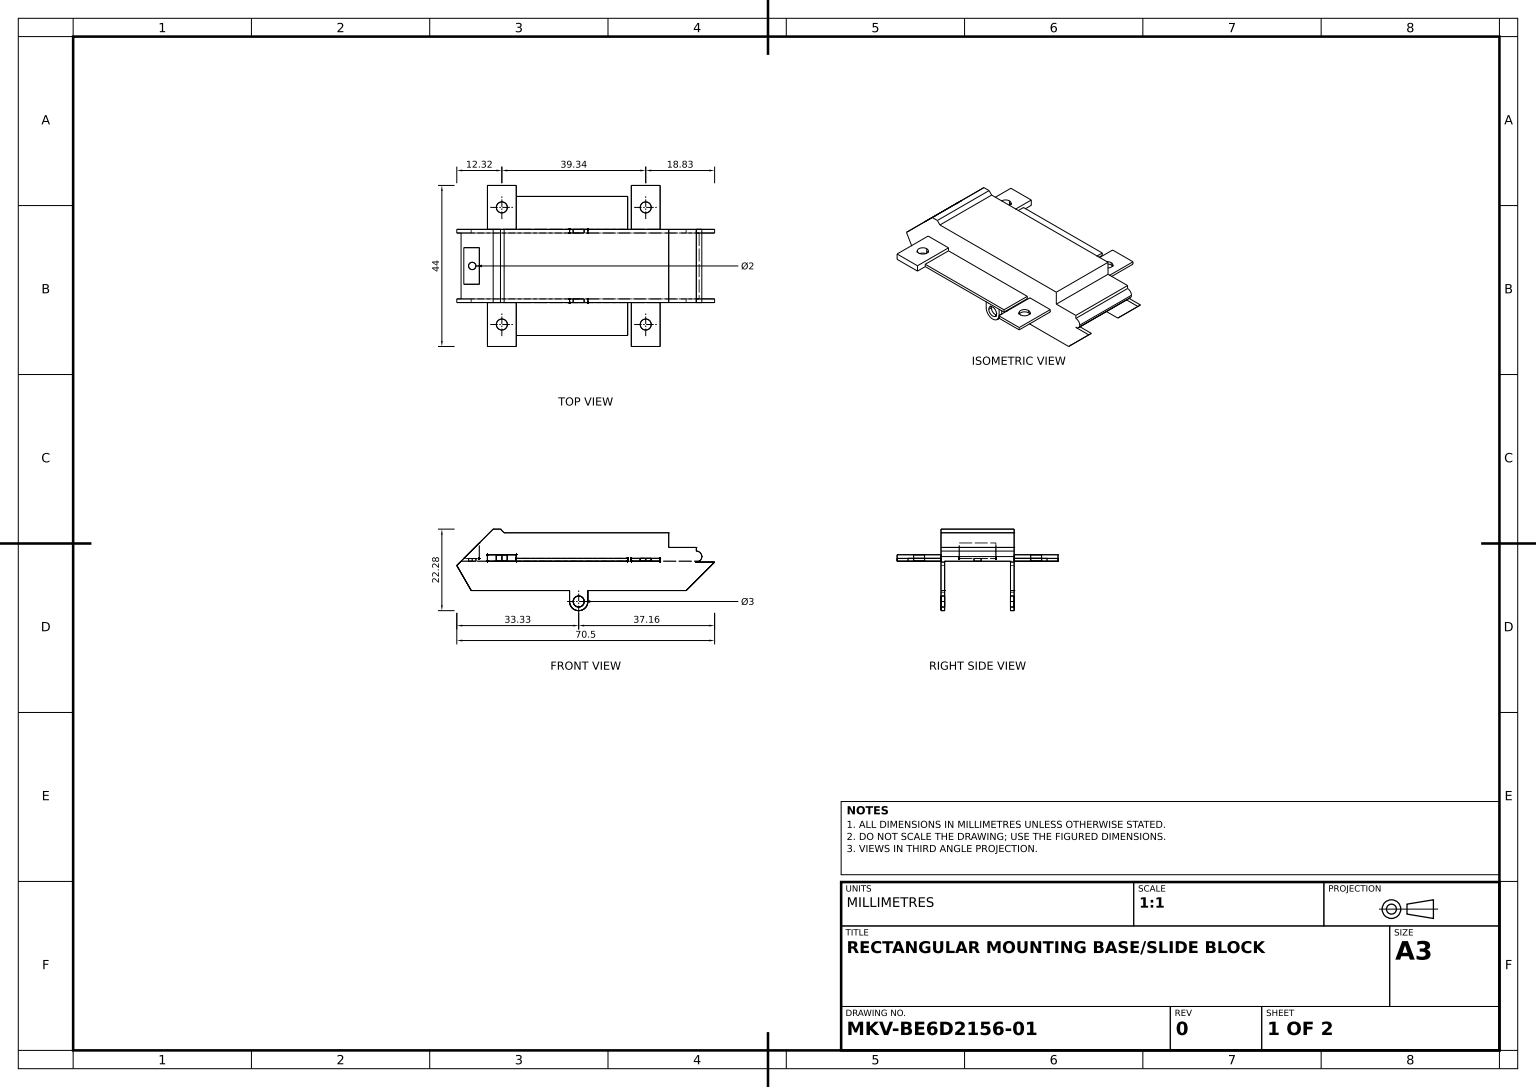
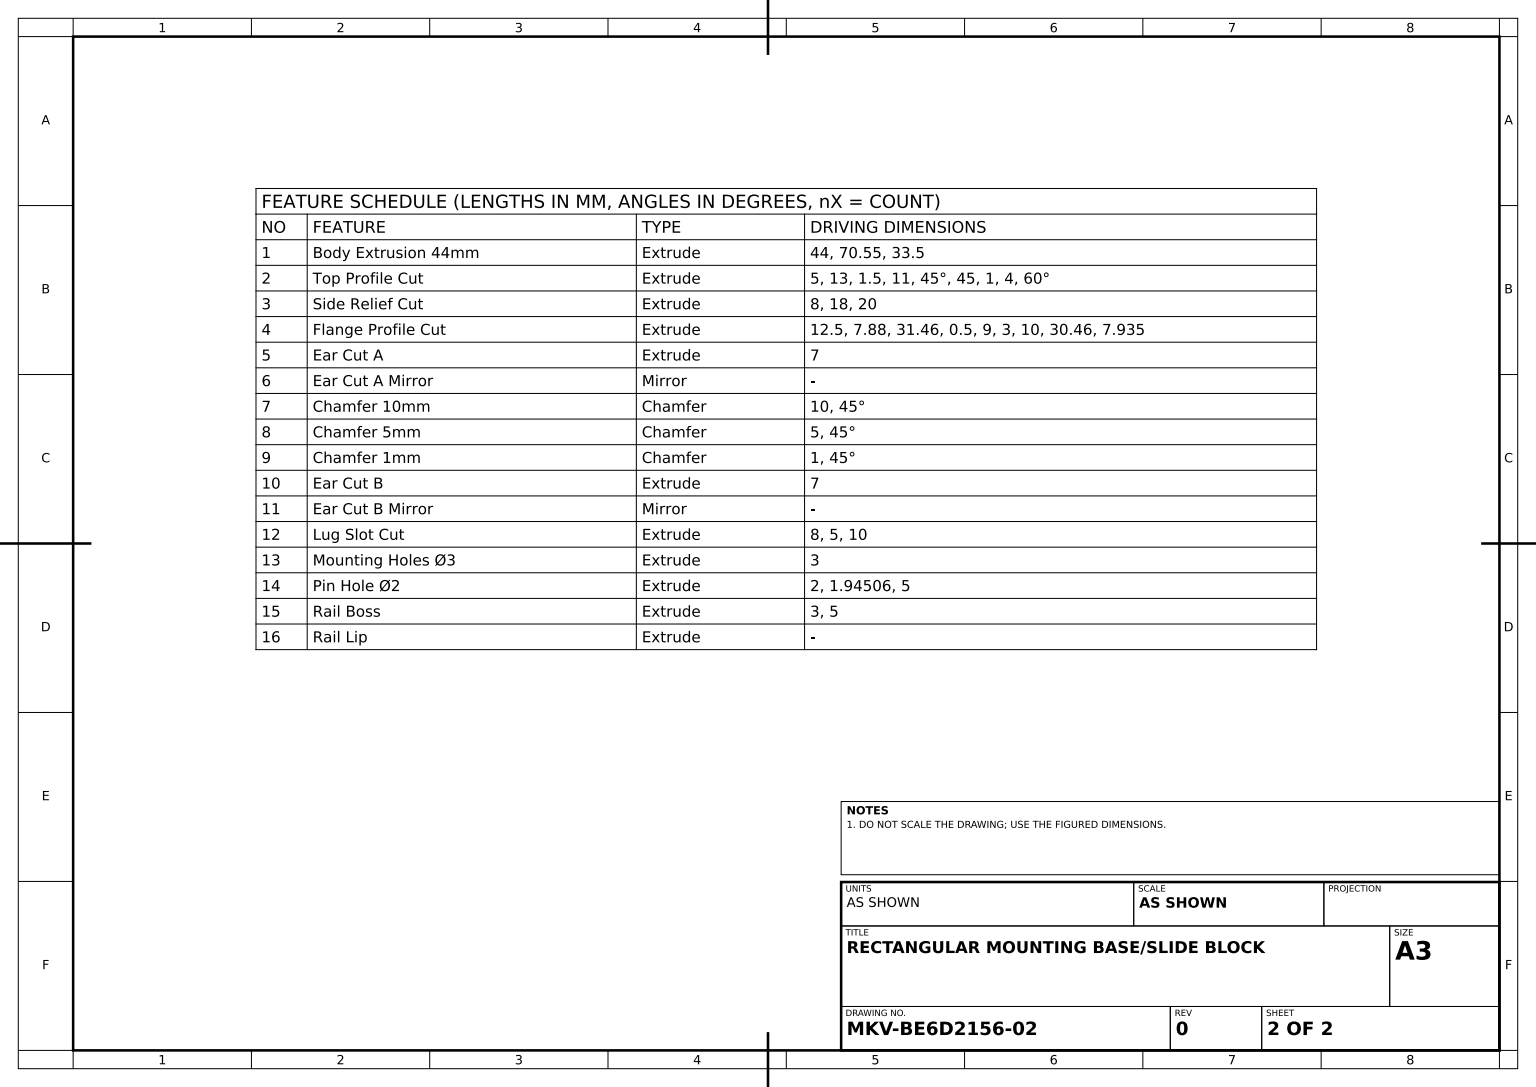
solid
v1 (-3.389087,-19.75,-10)
v2 (-0.389087,-19.75,-10)
e1 v1 v2 CIRCLE(AX(P(-1.889087,-19.75,-10),D(0,0,-1),D(-1,0,0)),1.5)
v3 (-0.389087,-19.75,-9)
e2 v3 v2 LINE
v4 (-3.389087,-19.75,-9)
e3 v3 v4 CIRCLE(AX(P(-1.889087,-19.75,-9),D(0,0,1),D(-1,0,0)),1.5)
e4 v4 v1 LINE
face CYL(AX(P(-1.889087,-19.75,-1.566966),D(0,0,-1),D(-1,0,0)),1.5) rev [e1 -e2 e3 e4]
v5 (22.725,-4.971825,-10)
v6 (22.725,-0.971825,-10)
e5 v5 v6 LINE
v7 (22.725,-0.971825,10)
e6 v6 v7 LINE
v8 (22.725,-4.971825,10)
e7 v8 v7 LINE
e8 v5 v8 LINE
face PLANE(AX(P(22.725,0,-22),D(-1,0,0),D(0,0,1))) rev [e5 e6 -e7 -e8]
v9 (35.275,-8.971825,9)
v10 (35.275,-8.971825,10)
e9 v9 v10 LINE
v11 (30.275,-8.971825,9)
e10 v11 v9 LINE
v12 (30.275,-8.971825,10)
e11 v11 v12 LINE
e12 v12 v10 LINE
face PLANE(AX(P(0,-8.971825,-22),D(0,-1,0),D(0,0,-1))) rev [-e9 -e10 e11 e12]
v13 (16.44,-8.75,-17.5)
v14 (16.44,-7.971825,-17.5)
e13 v13 v14 LINE
v15 (16.44,-7.971825,-14.5)
e14 v14 v15 CIRCLE(AX(P(16.44,-7.971825,-16),D(0,1,0),D(0,0,1)),1.5)
v16 (16.44,-8.75,-14.5)
e15 v16 v15 LINE
e16 v16 v13 CIRCLE(AX(P(16.44,-8.75,-16),D(0,-1,0),D(0,0,-1)),1.5)
face CYL(AX(P(16.44,-16.75,-16),D(0,1,0),D(0,0,1)),1.5) rev [e13 e14 -e15 e16]
v17 (20.38,-7.971825,22)
v18 (12.5,-7.971825,22)
e17 v17 v18 LINE
v19 (12.5,-8.75,22)
e18 v19 v18 LINE
v20 (20.38,-8.75,22)
e19 v19 v20 LINE
e20 v20 v17 LINE
face PLANE(AX(P(0,0,22),D(0,0,1),D(1,0,0))) [e17 -e18 e19 e20]
v21 (20.38,-8.75,10)
e21 v20 v21 LINE
v22 (20.38,-7.971825,10)
e22 v21 v22 LINE
e23 v22 v17 LINE
face PLANE(AX(P(20.38,-16.75,0),D(1,0,0),D(0,1,0))) [e21 e22 e23 -e20]
v23 (-30.998233,-8.75,-1)
v24 (-30.998233,-8.75,1)
e24 v23 v24 CIRCLE(AX(P(-30.998233,-8.75,0),D(0,-1,0),D(0,0,-1)),1)
v25 (-30.998233,-8,1)
e25 v24 v25 LINE
v26 (-30.998233,-8,-1)
e26 v25 v26 CIRCLE(AX(P(-30.998233,-8,0),D(0,1,0),D(0,0,1)),1)
e27 v23 v26 LINE
face CYL(AX(P(-30.998233,-16.75,0),D(0,1,0),D(0,0,1)),1) rev [e24 e25 e26 -e27]
v27 (27.496825,-16.75,10)
e28 v10 v27 LINE
v28 (27.496825,-16.75,9)
e29 v28 v27 LINE
e30 v9 v28 LINE
face PLANE(AX(P(22.123413,-22.123413,-22),D(-0.707106781,0.707106781,0),D(-0.707106781,-0.707106781,0))) rev [e9 e28 -e29 -e30]
v29 (-26.84,-8.75,10)
v30 (-26.84,-8.75,22)
e31 v29 v30 LINE
v31 (-26.84,-6.971825,22)
e32 v30 v31 LINE
v32 (-26.84,-6.971825,10)
e33 v31 v32 LINE
e34 v29 v32 LINE
face PLANE(AX(P(-26.84,-16.75,0),D(-1,0,0),D(0,-1,0))) [e31 e32 e33 -e34]
v33 (-22.9,-8.75,-17.5)
v34 (-22.9,-8.75,-14.5)
e35 v33 v34 CIRCLE(AX(P(-22.9,-8.75,-16),D(0,-1,0),D(0,0,-1)),1.5)
e36 v34 v33 CIRCLE(AX(P(-22.9,-8.75,-16),D(0,-1,0),D(0,0,-1)),1.5)
v35 (-18.96,-8.75,-19)
v36 (-18.96,-8.75,-22)
e37 v35 v36 LINE
v37 (11.5,-8.75,-19)
e38 v35 v37 LINE
v38 (11.5,-8.75,-10)
e39 v37 v38 LINE
v39 (-26.84,-8.75,-10)
e40 v39 v38 LINE
v40 (-26.84,-8.75,-22)
e41 v40 v39 LINE
e42 v40 v36 LINE
face PLANE(AX(P(-35.275,-8.75,-10),D(0,-1,0),D(0,0,-1))) [-e35 -e36] [-e37 e38 e39 -e40 -e41 e42]
e43 v26 v25 CIRCLE(AX(P(-30.998233,-8,0),D(0,1,0),D(0,0,1)),1)
v41 (-33.303175,-8,5)
v42 (-29.053175,-8,5)
e44 v41 v42 LINE
v43 (-29.053175,-8,-5)
e45 v42 v43 LINE
v44 (-33.303175,-8,-5)
e46 v43 v44 LINE
e47 v41 v44 LINE
face PLANE(AX(P(0,-8,0),D(0,1,0),D(0,0,1))) [-e43 -e26] [e44 e45 e46 -e47]
v45 (-31.275,-16.75,-10)
v46 (-4.389087,-16.75,-10)
e48 v45 v46 LINE
v47 (-4.389087,-16.75,-9)
e49 v47 v46 LINE
v48 (-31.275,-16.75,-9)
e50 v48 v47 LINE
e51 v45 v48 LINE
face PLANE(AX(P(-35.275,-16.75,22),D(0,1,0),D(0,0,1))) rev [e48 -e49 -e50 -e51]
v49 (-29.053175,-3.75,5)
e52 v42 v49 LINE
v50 (-29.053175,-3.75,-5)
e53 v49 v50 LINE
e54 v43 v50 LINE
face PLANE(AX(P(-29.053175,-8,-5),D(1,0,0),D(0,0,-1))) rev [e52 e53 -e54 -e45]
e55 v24 v23 CIRCLE(AX(P(-30.998233,-8.75,0),D(0,-1,0),D(0,0,-1)),1)
face CYL(AX(P(-30.998233,-16.75,0),D(0,1,0),D(0,0,1)),1) rev [e27 e43 -e25 e55]
v51 (-18.96,-6.971825,-10)
v52 (-18.96,-6.971825,-22)
e56 v51 v52 LINE
v53 (-26.84,-6.971825,-22)
e57 v52 v53 LINE
v54 (-26.84,-6.971825,-10)
e58 v53 v54 LINE
e59 v54 v51 LINE
v55 (-22.9,-6.971825,-17.5)
v56 (-22.9,-6.971825,-14.5)
e60 v55 v56 CIRCLE(AX(P(-22.9,-6.971825,-16),D(0,-1,0),D(1,0,0)),1.5)
e61 v56 v55 CIRCLE(AX(P(-22.9,-6.971825,-16),D(0,-1,0),D(1,0,0)),1.5)
face PLANE(AX(P(0,-6.971825,0),D(0,-1,0),D(1,0,0))) rev [e56 e57 e58 e59] [e60 e61]
v57 (11.5,-7.971825,10)
v58 (11.5,-7.971825,19)
e62 v57 v58 LINE
v59 (11.5,-8.75,19)
e63 v59 v58 LINE
v60 (11.5,-8.75,10)
e64 v60 v59 LINE
e65 v60 v57 LINE
face PLANE(AX(P(11.5,-16.75,0),D(-1,0,0),D(0,-1,0))) rev [e62 -e63 -e64 e65]
e66 v36 v52 LINE
v61 (-18.96,-7.971825,-10)
e67 v61 v51 LINE
v62 (-18.96,-7.971825,-19)
e68 v62 v61 LINE
e69 v35 v62 LINE
face PLANE(AX(P(-18.96,-16.75,0),D(-1,0,0),D(0,0,1))) rev [e66 -e56 -e67 -e68 -e69 e37]
e70 v34 v56 LINE
e71 v33 v55 LINE
face CYL(AX(P(-22.9,-16.75,-16),D(0,1,0),D(0,0,1)),1.5) rev [e35 e70 -e60 -e71]
v63 (-22.9,-8.75,17.5)
v64 (-22.9,-6.971825,17.5)
e72 v63 v64 LINE
v65 (-22.9,-8.75,14.5)
e73 v65 v63 CIRCLE(AX(P(-22.9,-8.75,16),D(0,1,0),D(0,0,1)),1.5)
v66 (-22.9,-6.971825,14.5)
e74 v65 v66 LINE
e75 v64 v66 CIRCLE(AX(P(-22.9,-6.971825,16),D(0,-1,0),D(1,0,0)),1.5)
face CYL(AX(P(-22.9,-16.75,16),D(0,1,0),D(0,0,1)),1.5) rev [-e72 -e73 e74 -e75]
v67 (12.5,-7.971825,10)
e76 v67 v22 LINE
e77 v18 v67 LINE
v68 (16.44,-7.971825,14.5)
v69 (16.44,-7.971825,17.5)
e78 v68 v69 CIRCLE(AX(P(16.44,-7.971825,16),D(0,1,0),D(0,0,1)),1.5)
e79 v69 v68 CIRCLE(AX(P(16.44,-7.971825,16),D(0,1,0),D(0,0,1)),1.5)
face PLANE(AX(P(0,-7.971825,0),D(0,1,0),D(0,0,-1))) [-e23 -e76 -e77 -e17] [-e78 -e79]
v70 (0.610913,-19.75,-9)
v71 (0.610913,-19.75,-10)
e80 v70 v71 LINE
v72 (0.610913,-16.75,-10)
e81 v72 v71 LINE
v73 (0.610913,-16.75,-9)
e82 v73 v72 LINE
e83 v70 v73 LINE
face PLANE(AX(P(0.610913,-19.75,-1.566966),D(1,0,0),D(0,1,0))) [e80 -e81 -e82 -e83]
v74 (-18.96,-7.971825,19)
e84 v58 v74 LINE
v75 (-18.96,-8.75,19)
e85 v75 v74 LINE
e86 v59 v75 LINE
face PLANE(AX(P(0,-16.75,19),D(0,0,-1),D(-1,0,0))) rev [e84 -e85 -e86 e63]
v76 (30.275,-4.971825,10)
e87 v76 v8 LINE
v77 (30.275,-4.971825,-10)
e88 v77 v76 LINE
e89 v77 v5 LINE
face PLANE(AX(P(0,-4.971825,-22),D(0,-1,0),D(0,0,-1))) rev [e8 -e87 -e88 e89]
v78 (0.610913,-16.75,10)
e90 v78 v27 LINE
v79 (0.610913,-16.75,9)
e91 v79 v78 LINE
e92 v79 v28 LINE
face PLANE(AX(P(-35.275,-16.75,22),D(0,1,0),D(0,0,1))) rev [-e90 -e91 e92 e29]
e93 v2 v1 CIRCLE(AX(P(-1.889087,-19.75,-10),D(0,0,-1),D(-1,0,0)),1.5)
e94 v4 v3 CIRCLE(AX(P(-1.889087,-19.75,-9),D(0,0,1),D(-1,0,0)),1.5)
face CYL(AX(P(-1.889087,-19.75,-1.566966),D(0,0,-1),D(-1,0,0)),1.5) rev [e2 e93 -e4 e94]
v80 (12.5,-8.75,10)
e95 v80 v67 LINE
e96 v80 v19 LINE
face PLANE(AX(P(12.5,-16.75,0),D(-1,0,0),D(0,-1,0))) [e77 -e95 e96 e18]
v81 (-35.220086,-9.916911,-9)
v82 (-35.220086,-9.916911,-10)
e97 v81 v82 LINE
e98 v45 v82 LINE
e99 v48 v81 LINE
face PLANE(AX(P(-30.709213,-17.729972,-22),D(0.866025404,0.5,0),D(-0.5,0.866025404,0))) rev [e97 -e98 e51 e99]
e100 v39 v54 LINE
e101 v40 v53 LINE
face PLANE(AX(P(-26.84,-16.75,0),D(1,0,0),D(0,1,0))) rev [e41 e100 -e58 -e101]
v83 (-4.389087,-19.75,-9)
e102 v83 v70 CIRCLE(AX(P(-1.889087,-19.75,-9),D(0,0,1),D(-1,0,0)),2.5)
v84 (-4.389087,-19.75,-10)
e103 v83 v84 LINE
e104 v71 v84 CIRCLE(AX(P(-1.889087,-19.75,-10),D(0,0,-1),D(-1,0,0)),2.5)
face CYL(AX(P(-1.889087,-19.75,-1.566966),D(0,0,-1),D(-1,0,0)),2.5) [-e80 -e102 e103 -e104]
v85 (11.5,-7.971825,-10)
e105 v61 v85 LINE
v86 (11.5,-7.971825,-19)
e106 v85 v86 LINE
e107 v86 v62 LINE
face PLANE(AX(P(0,-7.971825,0),D(0,-1,0),D(0,0,-1))) rev [e105 e106 e107 e68]
v87 (35.275,-8.971825,-9)
v88 (27.496825,-16.75,-9)
e108 v87 v88 LINE
v89 (30.275,-8.971825,-9)
e109 v89 v87 LINE
v90 (31.060028,-8.75,-9)
e110 v90 v89 CIRCLE(AX(P(30.275,-7.471825,-9),D(0,0,-1),D(-1,0,0)),1.5)
v91 (-34.053175,-8.75,-9)
e111 v91 v90 LINE
e112 v91 v81 LINE
e113 v47 v83 LINE
e114 v73 v88 LINE
face PLANE(AX(P(-35.275,-16.75,-9),D(0,0,-1),D(-1,0,0))) rev [-e108 -e109 -e110 -e111 e112 -e99 e50 e113 e102 e83 e114] [-e94 -e3]
v92 (-4.389087,-16.75,9)
v93 (-4.389087,-16.75,10)
e115 v92 v93 LINE
v94 (-4.389087,-19.75,9)
e116 v92 v94 LINE
v95 (-4.389087,-19.75,10)
e117 v94 v95 LINE
e118 v93 v95 LINE
face PLANE(AX(P(-4.389087,-16.75,1.566966),D(-1,0,0),D(0,0,1))) [-e115 e116 e117 -e118]
v96 (31.775,-7.471825,10)
e119 v96 v12 CIRCLE(AX(P(30.275,-7.471825,10),D(0,0,-1),D(-1,0,0)),1.5)
v97 (31.060028,-8.75,9)
e120 v97 v11 CIRCLE(AX(P(30.275,-7.471825,9),D(0,0,-1),D(-1,0,0)),1.5)
e121 v90 v97 LINE
v98 (30.275,-8.971825,-10)
e122 v98 v89 LINE
v99 (31.775,-7.471825,-10)
e123 v99 v98 CIRCLE(AX(P(30.275,-7.471825,-10),D(0,0,-1),D(-1,0,0)),1.5)
e124 v99 v96 LINE
face CYL(AX(P(30.275,-7.471825,-22),D(0,0,1),D(1,0,0)),1.5) [e119 -e11 -e120 -e121 e110 -e122 -e123 e124]
e125 v41 v49 LINE
face PLANE(AX(P(-34.053175,-8,5),D(0,0,1),D(1,0,0))) rev [-e44 e125 -e52]
v100 (12.5,-8.75,-22)
v101 (12.5,-7.971825,-22)
e126 v100 v101 LINE
v102 (12.5,-8.75,-10)
e127 v100 v102 LINE
v103 (12.5,-7.971825,-10)
e128 v102 v103 LINE
e129 v101 v103 LINE
face PLANE(AX(P(12.5,-16.75,0),D(1,0,0),D(0,1,0))) rev [-e126 e127 e128 -e129]
v104 (-22.275,-0.971825,-10)
v105 (-22.275,-0.971825,10)
e130 v104 v105 LINE
v106 (-23.275,0.028175,-10)
e131 v106 v104 LINE
v107 (-23.275,0.028175,10)
e132 v107 v106 LINE
e133 v107 v105 LINE
face PLANE(AX(P(-22.275,-0.971825,-22),D(-0.707106781,-0.707106781,0),D(0,0,1))) rev [-e130 -e131 -e132 e133]
v108 (35.275,-8.971825,-10)
e134 v108 v87 LINE
e135 v98 v108 LINE
face PLANE(AX(P(0,-8.971825,-22),D(0,-1,0),D(0,0,-1))) rev [e122 e109 -e134 -e135]
v109 (-18.96,-7.971825,10)
e136 v74 v109 LINE
e137 v109 v57 LINE
face PLANE(AX(P(0,-7.971825,0),D(0,-1,0),D(0,0,1))) rev [-e136 -e84 -e62 -e137]
v110 (-18.96,-8.75,22)
v111 (-18.96,-6.971825,22)
e138 v110 v111 LINE
e139 v110 v75 LINE
v112 (-18.96,-6.971825,10)
e140 v109 v112 LINE
e141 v112 v111 LINE
face PLANE(AX(P(-18.96,-16.75,0),D(1,0,0),D(0,0,-1))) [-e138 e139 e85 e136 e140 e141]
e142 v37 v86 LINE
e143 v38 v85 LINE
face PLANE(AX(P(11.5,-16.75,0),D(1,0,0),D(0,1,0))) [-e39 e142 -e106 -e143]
v113 (16.44,-8.75,17.5)
v114 (16.44,-8.75,14.5)
e144 v113 v114 CIRCLE(AX(P(16.44,-8.75,16),D(0,1,0),D(0,0,1)),1.5)
e145 v114 v113 CIRCLE(AX(P(16.44,-8.75,16),D(0,1,0),D(0,0,1)),1.5)
e146 v80 v21 LINE
face PLANE(AX(P(-35.275,-8.75,10),D(0,1,0),D(0,0,1))) rev [e144 e145] [e146 -e21 -e19 -e96]
e147 v111 v31 LINE
e148 v30 v110 LINE
face PLANE(AX(P(0,0,22),D(0,0,1),D(1,0,0))) [e138 e147 -e32 e148]
e149 v50 v44 LINE
face PLANE(AX(P(-34.053175,-8,-5),D(0,0,-1),D(-1,0,0))) rev [-e46 e54 e149]
e150 v84 v46 LINE
v115 (-25.275,0.028175,-10)
e151 v82 v115 LINE
e152 v115 v106 LINE
e153 v6 v104 LINE
v116 (30.275,-5.971825,-10)
e154 v116 v77 LINE
e155 v116 v99 CIRCLE(AX(P(30.275,-7.471825,-10),D(0,0,-1),D(-1,0,0)),1.5)
v117 (27.496825,-16.75,-10)
e156 v108 v117 LINE
e157 v72 v117 LINE
v118 (20.38,-7.971825,-10)
e158 v103 v118 LINE
v119 (20.38,-8.75,-10)
e159 v102 v119 LINE
e160 v119 v118 LINE
face PLANE(AX(P(-35.275,-16.75,-10),D(0,0,-1),D(-1,0,0))) [-e93 -e1] [e150 -e48 e98 e151 e152 e131 -e153 -e5 -e89 -e154 e155 e123 e135 e156 -e157 e81 e104] [-e100 e40 e143 -e105 e67 -e59] [-e158 -e128 e159 e160]
v120 (-34.053175,-8.75,9)
e161 v120 v91 LINE
v121 (-35.220086,-9.916911,9)
e162 v121 v120 LINE
v122 (-35.220086,-9.916911,10)
e163 v122 v121 LINE
v123 (-25.275,0.028175,10)
e164 v123 v122 LINE
e165 v115 v123 LINE
face PLANE(AX(P(-25.275,0.028175,-22),D(0.707106781,-0.707106781,0),D(0,0,1))) rev [-e149 -e53 -e125 e47] [-e112 -e161 -e162 -e163 -e164 -e165 -e151 -e97]
face CYL(AX(P(-22.9,-16.75,-16),D(0,1,0),D(0,0,1)),1.5) rev [e36 e71 -e61 -e70]
e166 v63 v65 CIRCLE(AX(P(-22.9,-8.75,16),D(0,1,0),D(0,0,1)),1.5)
e167 v66 v64 CIRCLE(AX(P(-22.9,-6.971825,16),D(0,-1,0),D(1,0,0)),1.5)
face CYL(AX(P(-22.9,-16.75,16),D(0,1,0),D(0,0,1)),1.5) rev [-e74 -e166 e72 -e167]
v124 (20.38,-8.75,-22)
e168 v100 v124 LINE
e169 v119 v124 LINE
e170 v13 v16 CIRCLE(AX(P(16.44,-8.75,-16),D(0,-1,0),D(0,0,-1)),1.5)
face PLANE(AX(P(-35.275,-8.75,-10),D(0,-1,0),D(0,0,-1))) [e168 -e169 -e159 -e127] [-e16 -e170]
e171 v117 v88 LINE
face PLANE(AX(P(22.123413,-22.123413,-22),D(-0.707106781,0.707106781,0),D(-0.707106781,-0.707106781,0))) rev [-e156 e134 e108 -e171]
e172 v113 v69 LINE
e173 v114 v68 LINE
face CYL(AX(P(16.44,-16.75,16),D(0,1,0),D(0,0,1)),1.5) rev [-e144 e172 e79 -e173]
v125 (20.38,-7.971825,-22)
e174 v125 v101 LINE
e175 v124 v125 LINE
face PLANE(AX(P(0,0,-22),D(0,0,1),D(1,0,0))) rev [e126 -e174 -e175 -e168]
e176 v7 v105 LINE
face PLANE(AX(P(0,-0.971825,-22),D(0,-1,0),D(0,0,-1))) rev [e130 -e176 -e6 e153]
v126 (-31.275,-16.75,10)
e177 v126 v93 LINE
v127 (-31.275,-16.75,9)
e178 v127 v126 LINE
e179 v127 v92 LINE
face PLANE(AX(P(-35.275,-16.75,22),D(0,1,0),D(0,0,1))) rev [-e177 -e178 e179 e115]
e180 v120 v97 LINE
face PLANE(AX(P(-35.275,-8.75,9),D(0,-1,0),D(0,0,-1))) [-e55 -e24] [e121 -e180 e161 e111]
face CYL(AX(P(16.44,-16.75,16),D(0,1,0),D(0,0,1)),1.5) rev [e173 e78 -e172 -e145]
e181 v123 v107 LINE
face PLANE(AX(P(0,0.028175,-22),D(0,-1,0),D(1,0,0))) rev [e165 e181 e132 -e152]
e182 v127 v121 LINE
e183 v126 v122 LINE
face PLANE(AX(P(-30.709213,-17.729972,-22),D(0.866025404,0.5,0),D(-0.5,0.866025404,0))) rev [-e182 e178 e183 e163]
e184 v29 v60 LINE
face PLANE(AX(P(-35.275,-8.75,10),D(0,1,0),D(0,0,1))) rev [e184 e64 e86 -e139 -e148 -e31] [e166 e73]
face PLANE(AX(P(0,0,-22),D(0,0,1),D(1,0,0))) rev [-e66 -e42 e101 -e57]
face PLANE(AX(P(-4.389087,-16.75,-1.566966),D(-1,0,0),D(0,0,1))) [-e113 e49 -e150 -e103]
face PLANE(AX(P(-35.275,-16.75,22),D(0,1,0),D(0,0,1))) rev [e171 -e114 e82 e157]
v128 (-0.389087,-19.75,9)
v129 (-0.389087,-19.75,10)
e185 v128 v129 LINE
v130 (-3.389087,-19.75,9)
e186 v130 v128 CIRCLE(AX(P(-1.889087,-19.75,9),D(0,0,1),D(-1,0,0)),1.5)
v131 (-3.389087,-19.75,10)
e187 v130 v131 LINE
e188 v131 v129 CIRCLE(AX(P(-1.889087,-19.75,10),D(0,0,1),D(1,0,0)),1.5)
face CYL(AX(P(-1.889087,-19.75,1.566966),D(0,0,1),D(1,0,0)),1.5) rev [-e185 -e186 e187 e188]
e189 v118 v125 LINE
e190 v15 v14 CIRCLE(AX(P(16.44,-7.971825,-16),D(0,1,0),D(0,0,1)),1.5)
face PLANE(AX(P(0,-7.971825,0),D(0,1,0),D(0,0,1))) [e129 e158 e189 e174] [-e14 -e190]
face CYL(AX(P(16.44,-16.75,-16),D(0,1,0),D(0,0,1)),1.5) rev [e190 -e13 e170 e15]
e191 v32 v112 LINE
face PLANE(AX(P(0,-6.971825,0),D(0,-1,0),D(1,0,0))) rev [-e147 -e141 -e191 -e33] [e75 e167]
v132 (30.275,-5.971825,10)
e192 v116 v132 LINE
e193 v132 v76 LINE
face PLANE(AX(P(30.275,0,-22),D(-1,0,0),D(0,0,1))) rev [-e192 e154 e88 -e193]
v133 (0.610913,-19.75,9)
v134 (0.610913,-19.75,10)
e194 v133 v134 LINE
e195 v95 v134 CIRCLE(AX(P(-1.889087,-19.75,10),D(0,0,1),D(1,0,0)),2.5)
e196 v94 v133 CIRCLE(AX(P(-1.889087,-19.75,9),D(0,0,1),D(-1,0,0)),2.5)
face CYL(AX(P(-1.889087,-19.75,1.566966),D(0,0,1),D(1,0,0)),2.5) [e194 -e195 -e117 e196]
face PLANE(AX(P(0,-16.75,-19),D(0,0,-1),D(-1,0,0))) [-e142 -e38 e69 -e107]
face PLANE(AX(P(20.38,-16.75,0),D(-1,0,0),D(0,-1,0))) rev [-e189 -e160 e169 e175]
e197 v128 v130 CIRCLE(AX(P(-1.889087,-19.75,9),D(0,0,1),D(-1,0,0)),1.5)
e198 v133 v79 LINE
face PLANE(AX(P(-35.275,-16.75,9),D(0,0,-1),D(-1,0,0))) [e186 e197] [-e92 -e198 -e196 -e116 -e179 e182 e162 e180 e120 e10 e30]
e199 v129 v131 CIRCLE(AX(P(-1.889087,-19.75,10),D(0,0,1),D(1,0,0)),1.5)
e200 v134 v78 LINE
e201 v132 v96 CIRCLE(AX(P(30.275,-7.471825,10),D(0,0,-1),D(-1,0,0)),1.5)
face PLANE(AX(P(-35.275,-16.75,10),D(0,0,-1),D(-1,0,0))) rev [-e188 -e199] [-e65 -e184 e34 e191 -e140 e137] [-e146 e95 e76 -e22] [-e183 e177 e118 e195 e200 e90 -e28 -e12 -e119 -e201 e193 e87 e7 e176 -e133 -e181 e164]
face CYL(AX(P(-1.889087,-19.75,1.566966),D(0,0,1),D(1,0,0)),1.5) rev [-e197 e185 e199 -e187]
face PLANE(AX(P(0.610913,-16.75,1.566966),D(1,0,0),D(0,1,0))) [e198 e91 -e200 -e194]
face CYL(AX(P(30.275,-7.471825,-22),D(0,0,1),D(1,0,0)),1.5) [e192 e201 -e124 -e155]
